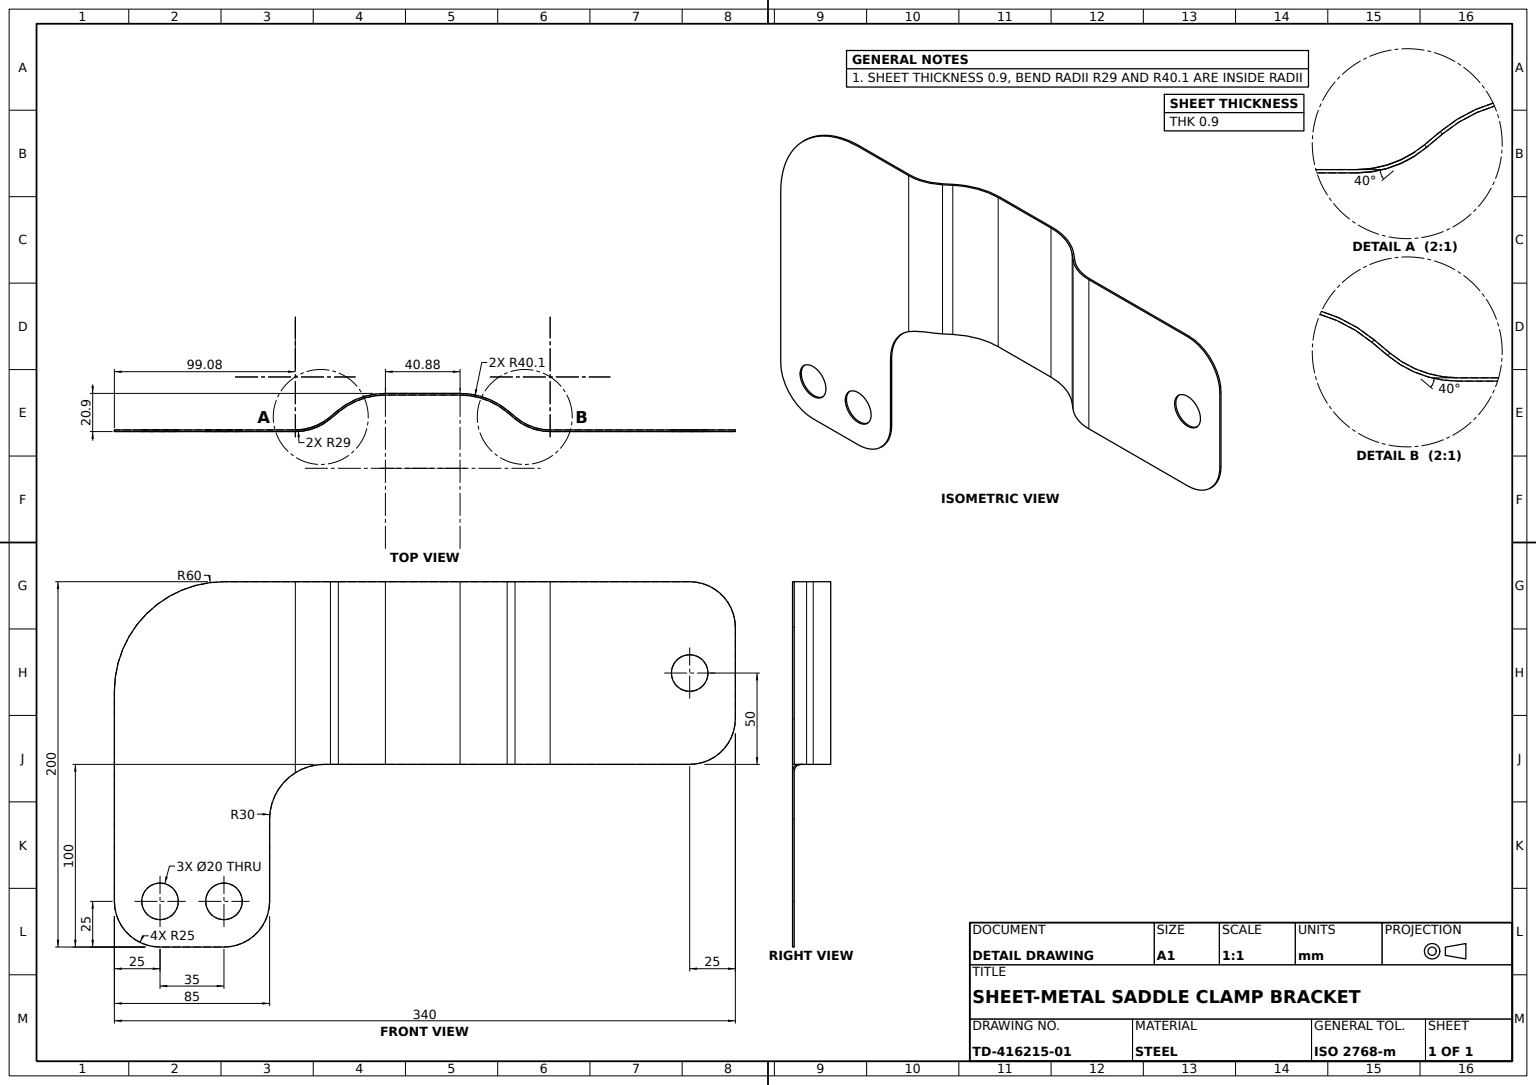
ISO-10303-21;
HEADER;
FILE_DESCRIPTION((''),'2;1');
FILE_NAME('','',(''),(''),'','','');
FILE_SCHEMA(('AUTOMOTIVE_DESIGN'));
ENDSEC;
DATA;
#1=APPLICATION_CONTEXT('');
#2=PRODUCT_CONTEXT('',#1,'mechanical');
#3=PRODUCT('','','',(#2));
#4=PRODUCT_DEFINITION_FORMATION('','',#3);
#5=PRODUCT_DEFINITION_CONTEXT('',#1,'design');
#6=PRODUCT_DEFINITION('','',#4,#5);
#7=PRODUCT_DEFINITION_SHAPE('','',#6);
#8=(LENGTH_UNIT()NAMED_UNIT(*)SI_UNIT(.MILLI.,.METRE.));
#9=(NAMED_UNIT(*)PLANE_ANGLE_UNIT()SI_UNIT($,.RADIAN.));
#10=(NAMED_UNIT(*)SI_UNIT($,.STERADIAN.)SOLID_ANGLE_UNIT());
#11=UNCERTAINTY_MEASURE_WITH_UNIT(LENGTH_MEASURE(1.E-05),#8,'distance_accuracy_value','');
#12=(GEOMETRIC_REPRESENTATION_CONTEXT(3)GLOBAL_UNCERTAINTY_ASSIGNED_CONTEXT((#11))GLOBAL_UNIT_ASSIGNED_CONTEXT((#8,#9,#10))REPRESENTATION_CONTEXT('',''));
#13=CARTESIAN_POINT('',(148.393881,0.,-221.));
#14=VERTEX_POINT('',#13);
#15=CARTESIAN_POINT('',(189.276262,0.,-221.));
#16=VERTEX_POINT('',#15);
#17=DIRECTION('',(1.,0.,0.));
#18=VECTOR('',#17,1000.);
#19=LINE('',#13,#18);
#20=EDGE_CURVE('',#14,#16,#19,.T.);
#21=ORIENTED_EDGE('',*,*,#20,.T.);
#22=CARTESIAN_POINT('',(189.276262,0.,-220.1));
#23=VERTEX_POINT('',#22);
#24=DIRECTION('',(0.,0.,-1.));
#25=VECTOR('',#24,1000.);
#26=LINE('',#15,#25);
#27=EDGE_CURVE('',#23,#16,#26,.T.);
#28=ORIENTED_EDGE('',*,*,#27,.F.);
#29=CARTESIAN_POINT('',(148.393881,0.,-220.1));
#30=VERTEX_POINT('',#29);
#31=LINE('',#29,#18);
#32=EDGE_CURVE('',#30,#23,#31,.T.);
#33=ORIENTED_EDGE('',*,*,#32,.F.);
#34=LINE('',#13,#25);
#35=EDGE_CURVE('',#30,#14,#34,.T.);
#36=ORIENTED_EDGE('',*,*,#35,.T.);
#37=EDGE_LOOP('',(#21,#28,#33,#36));
#38=FACE_OUTER_BOUND('',#37,.T.);
#39=DIRECTION('',(0.,-1.,0.));
#40=AXIS2_PLACEMENT_3D('',#13,#39,#17);
#41=PLANE('',#40);
#42=ADVANCED_FACE('',(#38),#41,.T.);
#43=CARTESIAN_POINT('',(60.,-100.,-201.));
#44=VERTEX_POINT('',#43);
#45=CARTESIAN_POINT('',(60.,-100.,-200.1));
#46=VERTEX_POINT('',#45);
#47=DIRECTION('',(0.,0.,1.));
#48=VECTOR('',#47,1000.);
#49=LINE('',#43,#48);
#50=EDGE_CURVE('',#44,#46,#49,.T.);
#51=ORIENTED_EDGE('',*,*,#50,.F.);
#52=CARTESIAN_POINT('',(85.,-75.,-201.));
#53=VERTEX_POINT('',#52);
#54=CARTESIAN_POINT('',(60.,-75.,-201.));
#55=AXIS2_PLACEMENT_3D('',#54,#24,#17);
#56=CIRCLE('',#55,25.);
#57=EDGE_CURVE('',#53,#44,#56,.T.);
#58=ORIENTED_EDGE('',*,*,#57,.F.);
#59=CARTESIAN_POINT('',(85.,-75.,-200.1));
#60=VERTEX_POINT('',#59);
#61=LINE('',#52,#25);
#62=EDGE_CURVE('',#60,#53,#61,.T.);
#63=ORIENTED_EDGE('',*,*,#62,.F.);
#64=CARTESIAN_POINT('',(60.,-75.,-200.1));
#65=AXIS2_PLACEMENT_3D('',#64,#47,#17);
#66=CIRCLE('',#65,25.);
#67=EDGE_CURVE('',#46,#60,#66,.T.);
#68=ORIENTED_EDGE('',*,*,#67,.F.);
#69=EDGE_LOOP('',(#51,#58,#63,#68));
#70=FACE_OUTER_BOUND('',#69,.T.);
#71=AXIS2_PLACEMENT_3D('',#54,#47,#17);
#72=CYLINDRICAL_SURFACE('',#71,25.);
#73=ADVANCED_FACE('',(#70),#72,.T.);
#74=CARTESIAN_POINT('',(215.052046,100.,-210.718382));
#75=VERTEX_POINT('',#74);
#76=CARTESIAN_POINT('',(215.630554,100.,-211.407822));
#77=VERTEX_POINT('',#76);
#78=DIRECTION('',(0.64278761,0.,-0.766044443));
#79=VECTOR('',#78,1000.);
#80=LINE('',#76,#79);
#81=EDGE_CURVE('',#75,#77,#80,.T.);
#82=ORIENTED_EDGE('',*,*,#81,.T.);
#83=CARTESIAN_POINT('',(189.276262,100.,-221.));
#84=VERTEX_POINT('',#83);
#85=CARTESIAN_POINT('',(189.276262,100.,-180.));
#86=DIRECTION('',(0.,1.,0.));
#87=AXIS2_PLACEMENT_3D('',#85,#86,#24);
#88=CIRCLE('',#87,41.);
#89=EDGE_CURVE('',#77,#84,#88,.T.);
#90=ORIENTED_EDGE('',*,*,#89,.T.);
#91=CARTESIAN_POINT('',(189.276262,100.,-220.1));
#92=VERTEX_POINT('',#91);
#93=LINE('',#83,#25);
#94=EDGE_CURVE('',#92,#84,#93,.T.);
#95=ORIENTED_EDGE('',*,*,#94,.F.);
#96=CIRCLE('',#87,40.1);
#97=EDGE_CURVE('',#75,#92,#96,.T.);
#98=ORIENTED_EDGE('',*,*,#97,.F.);
#99=EDGE_LOOP('',(#82,#90,#95,#98));
#100=FACE_OUTER_BOUND('',#99,.T.);
#101=AXIS2_PLACEMENT_3D('',#85,#86,#47);
#102=PLANE('',#101);
#103=ADVANCED_FACE('',(#100),#102,.T.);
#104=CARTESIAN_POINT('',(25.,-100.,-201.));
#105=VERTEX_POINT('',#104);
#106=CARTESIAN_POINT('',(99.080893,-100.,-201.));
#107=DIRECTION('',(-1.,0.,0.));
#108=VECTOR('',#107,1000.);
#109=LINE('',#106,#108);
#110=EDGE_CURVE('',#44,#105,#109,.T.);
#111=ORIENTED_EDGE('',*,*,#110,.F.);
#112=ORIENTED_EDGE('',*,*,#50,.T.);
#113=CARTESIAN_POINT('',(25.,-100.,-200.1));
#114=VERTEX_POINT('',#113);
#115=CARTESIAN_POINT('',(0.,-100.,-200.1));
#116=LINE('',#115,#108);
#117=EDGE_CURVE('',#46,#114,#116,.T.);
#118=ORIENTED_EDGE('',*,*,#117,.T.);
#119=LINE('',#104,#25);
#120=EDGE_CURVE('',#114,#105,#119,.T.);
#121=ORIENTED_EDGE('',*,*,#120,.T.);
#122=EDGE_LOOP('',(#111,#112,#118,#121));
#123=FACE_OUTER_BOUND('',#122,.T.);
#124=AXIS2_PLACEMENT_3D('',#106,#86,#107);
#125=PLANE('',#124);
#126=ADVANCED_FACE('',(#123),#125,.F.);
#127=CARTESIAN_POINT('',(315.,100.,-200.1));
#128=VERTEX_POINT('',#127);
#129=CARTESIAN_POINT('',(238.589251,100.,-200.1));
#130=VERTEX_POINT('',#129);
#131=LINE('',#129,#108);
#132=EDGE_CURVE('',#128,#130,#131,.T.);
#133=ORIENTED_EDGE('',*,*,#132,.T.);
#134=CARTESIAN_POINT('',(238.589251,0.,-200.1));
#135=VERTEX_POINT('',#134);
#136=VECTOR('',#39,1000.);
#137=LINE('',#129,#136);
#138=EDGE_CURVE('',#130,#135,#137,.T.);
#139=ORIENTED_EDGE('',*,*,#138,.T.);
#140=CARTESIAN_POINT('',(315.,0.,-200.1));
#141=VERTEX_POINT('',#140);
#142=LINE('',#134,#18);
#143=EDGE_CURVE('',#135,#141,#142,.T.);
#144=ORIENTED_EDGE('',*,*,#143,.T.);
#145=CARTESIAN_POINT('',(340.,25.,-200.1));
#146=VERTEX_POINT('',#145);
#147=CARTESIAN_POINT('',(315.,25.,-200.1));
#148=AXIS2_PLACEMENT_3D('',#147,#47,#17);
#149=CIRCLE('',#148,25.);
#150=EDGE_CURVE('',#141,#146,#149,.T.);
#151=ORIENTED_EDGE('',*,*,#150,.T.);
#152=CARTESIAN_POINT('',(340.,75.,-200.1));
#153=VERTEX_POINT('',#152);
#154=CARTESIAN_POINT('',(340.,100.,-200.1));
#155=LINE('',#154,#136);
#156=EDGE_CURVE('',#153,#146,#155,.T.);
#157=ORIENTED_EDGE('',*,*,#156,.F.);
#158=CARTESIAN_POINT('',(315.,75.,-200.1));
#159=AXIS2_PLACEMENT_3D('',#158,#47,#17);
#160=CIRCLE('',#159,25.);
#161=EDGE_CURVE('',#153,#128,#160,.T.);
#162=ORIENTED_EDGE('',*,*,#161,.T.);
#163=EDGE_LOOP('',(#133,#139,#144,#151,#157,#162));
#164=FACE_OUTER_BOUND('',#163,.T.);
#165=CARTESIAN_POINT('',(325.,50.,-200.1));
#166=VERTEX_POINT('',#165);
#167=CARTESIAN_POINT('',(305.,50.,-200.1));
#168=VERTEX_POINT('',#167);
#169=CARTESIAN_POINT('',(315.,50.,-200.1));
#170=AXIS2_PLACEMENT_3D('',#169,#47,#17);
#171=CIRCLE('',#170,10.);
#172=EDGE_CURVE('',#166,#168,#171,.T.);
#173=ORIENTED_EDGE('',*,*,#172,.F.);
#174=EDGE_CURVE('',#168,#166,#171,.T.);
#175=ORIENTED_EDGE('',*,*,#174,.F.);
#176=EDGE_LOOP('',(#173,#175));
#177=FACE_BOUND('',#176,.T.);
#178=AXIS2_PLACEMENT_3D('',#129,#47,#17);
#179=PLANE('',#178);
#180=ADVANCED_FACE('',(#164,#177),#179,.T.);
#181=CARTESIAN_POINT('',(305.,50.,-201.));
#182=VERTEX_POINT('',#181);
#183=CARTESIAN_POINT('',(305.,50.,44.));
#184=LINE('',#183,#25);
#185=EDGE_CURVE('',#168,#182,#184,.T.);
#186=ORIENTED_EDGE('',*,*,#185,.F.);
#187=ORIENTED_EDGE('',*,*,#174,.T.);
#188=CARTESIAN_POINT('',(325.,50.,-201.));
#189=VERTEX_POINT('',#188);
#190=CARTESIAN_POINT('',(325.,50.,44.));
#191=LINE('',#190,#25);
#192=EDGE_CURVE('',#166,#189,#191,.T.);
#193=ORIENTED_EDGE('',*,*,#192,.T.);
#194=CARTESIAN_POINT('',(315.,50.,-201.));
#195=AXIS2_PLACEMENT_3D('',#194,#24,#107);
#196=CIRCLE('',#195,10.);
#197=EDGE_CURVE('',#189,#182,#196,.T.);
#198=ORIENTED_EDGE('',*,*,#197,.T.);
#199=EDGE_LOOP('',(#186,#187,#193,#198));
#200=FACE_OUTER_BOUND('',#199,.T.);
#201=CARTESIAN_POINT('',(315.,50.,44.));
#202=AXIS2_PLACEMENT_3D('',#201,#24,#107);
#203=CYLINDRICAL_SURFACE('',#202,10.);
#204=ADVANCED_FACE('',(#200),#203,.F.);
#205=CARTESIAN_POINT('',(219.369901,0.,-207.095271));
#206=VERTEX_POINT('',#205);
#207=CARTESIAN_POINT('',(219.94841,0.,-207.784711));
#208=VERTEX_POINT('',#207);
#209=LINE('',#207,#79);
#210=EDGE_CURVE('',#206,#208,#209,.T.);
#211=ORIENTED_EDGE('',*,*,#210,.F.);
#212=CARTESIAN_POINT('',(215.052046,0.,-210.718382));
#213=VERTEX_POINT('',#212);
#214=DIRECTION('',(0.766044443,0.,0.64278761));
#215=VECTOR('',#214,1000.);
#216=LINE('',#212,#215);
#217=EDGE_CURVE('',#213,#206,#216,.T.);
#218=ORIENTED_EDGE('',*,*,#217,.F.);
#219=CARTESIAN_POINT('',(215.630554,0.,-211.407822));
#220=VERTEX_POINT('',#219);
#221=LINE('',#219,#79);
#222=EDGE_CURVE('',#213,#220,#221,.T.);
#223=ORIENTED_EDGE('',*,*,#222,.T.);
#224=LINE('',#219,#215);
#225=EDGE_CURVE('',#220,#208,#224,.T.);
#226=ORIENTED_EDGE('',*,*,#225,.T.);
#227=EDGE_LOOP('',(#211,#218,#223,#226));
#228=FACE_OUTER_BOUND('',#227,.T.);
#229=AXIS2_PLACEMENT_3D('',#219,#39,#214);
#230=PLANE('',#229);
#231=ADVANCED_FACE('',(#228),#230,.T.);
#232=CARTESIAN_POINT('',(0.,40.,-200.1));
#233=VERTEX_POINT('',#232);
#234=CARTESIAN_POINT('',(0.,40.,-201.));
#235=VERTEX_POINT('',#234);
#236=LINE('',#234,#25);
#237=EDGE_CURVE('',#233,#235,#236,.T.);
#238=ORIENTED_EDGE('',*,*,#237,.F.);
#239=CARTESIAN_POINT('',(60.,100.,-200.1));
#240=VERTEX_POINT('',#239);
#241=CARTESIAN_POINT('',(60.,40.,-200.1));
#242=AXIS2_PLACEMENT_3D('',#241,#47,#17);
#243=CIRCLE('',#242,60.);
#244=EDGE_CURVE('',#240,#233,#243,.T.);
#245=ORIENTED_EDGE('',*,*,#244,.F.);
#246=CARTESIAN_POINT('',(60.,100.,-201.));
#247=VERTEX_POINT('',#246);
#248=LINE('',#246,#48);
#249=EDGE_CURVE('',#247,#240,#248,.T.);
#250=ORIENTED_EDGE('',*,*,#249,.F.);
#251=CARTESIAN_POINT('',(60.,40.,-201.));
#252=AXIS2_PLACEMENT_3D('',#251,#24,#17);
#253=CIRCLE('',#252,60.);
#254=EDGE_CURVE('',#235,#247,#253,.T.);
#255=ORIENTED_EDGE('',*,*,#254,.F.);
#256=EDGE_LOOP('',(#238,#245,#250,#255));
#257=FACE_OUTER_BOUND('',#256,.T.);
#258=AXIS2_PLACEMENT_3D('',#251,#24,#107);
#259=CYLINDRICAL_SURFACE('',#258,60.);
#260=ADVANCED_FACE('',(#257),#259,.T.);
#261=CARTESIAN_POINT('',(118.300243,100.,-207.095271));
#262=VERTEX_POINT('',#261);
#263=CARTESIAN_POINT('',(118.300243,0.,-207.095271));
#264=VERTEX_POINT('',#263);
#265=LINE('',#261,#136);
#266=EDGE_CURVE('',#262,#264,#265,.T.);
#267=ORIENTED_EDGE('',*,*,#266,.T.);
#268=CARTESIAN_POINT('',(122.618098,0.,-210.718382));
#269=VERTEX_POINT('',#268);
#270=DIRECTION('',(0.766044443,0.,-0.64278761));
#271=VECTOR('',#270,1000.);
#272=LINE('',#263,#271);
#273=EDGE_CURVE('',#264,#269,#272,.T.);
#274=ORIENTED_EDGE('',*,*,#273,.T.);
#275=CARTESIAN_POINT('',(122.618098,100.,-210.718382));
#276=VERTEX_POINT('',#275);
#277=LINE('',#275,#136);
#278=EDGE_CURVE('',#276,#269,#277,.T.);
#279=ORIENTED_EDGE('',*,*,#278,.F.);
#280=DIRECTION('',(-0.766044443,0.,0.64278761));
#281=VECTOR('',#280,1000.);
#282=LINE('',#261,#281);
#283=EDGE_CURVE('',#276,#262,#282,.T.);
#284=ORIENTED_EDGE('',*,*,#283,.T.);
#285=EDGE_LOOP('',(#267,#274,#279,#284));
#286=FACE_OUTER_BOUND('',#285,.T.);
#287=DIRECTION('',(0.64278761,0.,0.766044443));
#288=AXIS2_PLACEMENT_3D('',#261,#287,#270);
#289=PLANE('',#288);
#290=ADVANCED_FACE('',(#286),#289,.T.);
#291=ORIENTED_EDGE('',*,*,#225,.F.);
#292=LINE('',#76,#136);
#293=EDGE_CURVE('',#77,#220,#292,.T.);
#294=ORIENTED_EDGE('',*,*,#293,.F.);
#295=CARTESIAN_POINT('',(219.94841,100.,-207.784711));
#296=VERTEX_POINT('',#295);
#297=CARTESIAN_POINT('',(138.081545,100.,-276.479167));
#298=DIRECTION('',(-0.766044443,0.,-0.64278761));
#299=VECTOR('',#298,1000.);
#300=LINE('',#297,#299);
#301=EDGE_CURVE('',#296,#77,#300,.T.);
#302=ORIENTED_EDGE('',*,*,#301,.F.);
#303=LINE('',#295,#136);
#304=EDGE_CURVE('',#296,#208,#303,.T.);
#305=ORIENTED_EDGE('',*,*,#304,.T.);
#306=EDGE_LOOP('',(#291,#294,#302,#305));
#307=FACE_OUTER_BOUND('',#306,.T.);
#308=DIRECTION('',(-0.64278761,0.,0.766044443));
#309=AXIS2_PLACEMENT_3D('',#76,#308,#214);
#310=PLANE('',#309);
#311=ADVANCED_FACE('',(#307),#310,.F.);
#312=CARTESIAN_POINT('',(315.,100.,-201.));
#313=VERTEX_POINT('',#312);
#314=LINE('',#312,#25);
#315=EDGE_CURVE('',#128,#313,#314,.T.);
#316=ORIENTED_EDGE('',*,*,#315,.F.);
#317=ORIENTED_EDGE('',*,*,#161,.F.);
#318=CARTESIAN_POINT('',(340.,75.,-201.));
#319=VERTEX_POINT('',#318);
#320=LINE('',#318,#48);
#321=EDGE_CURVE('',#319,#153,#320,.T.);
#322=ORIENTED_EDGE('',*,*,#321,.F.);
#323=CARTESIAN_POINT('',(315.,75.,-201.));
#324=AXIS2_PLACEMENT_3D('',#323,#24,#17);
#325=CIRCLE('',#324,25.);
#326=EDGE_CURVE('',#313,#319,#325,.T.);
#327=ORIENTED_EDGE('',*,*,#326,.F.);
#328=EDGE_LOOP('',(#316,#317,#322,#327));
#329=FACE_OUTER_BOUND('',#328,.T.);
#330=AXIS2_PLACEMENT_3D('',#323,#47,#17);
#331=CYLINDRICAL_SURFACE('',#330,25.);
#332=ADVANCED_FACE('',(#329),#331,.T.);
#333=CARTESIAN_POINT('',(238.589251,0.,-230.));
#334=AXIS2_PLACEMENT_3D('',#333,#86,#24);
#335=CIRCLE('',#334,29.9);
#336=EDGE_CURVE('',#206,#135,#335,.T.);
#337=ORIENTED_EDGE('',*,*,#336,.F.);
#338=ORIENTED_EDGE('',*,*,#210,.T.);
#339=CARTESIAN_POINT('',(238.589251,0.,-201.));
#340=VERTEX_POINT('',#339);
#341=AXIS2_PLACEMENT_3D('',#333,#86,#17);
#342=CIRCLE('',#341,29.);
#343=EDGE_CURVE('',#208,#340,#342,.T.);
#344=ORIENTED_EDGE('',*,*,#343,.T.);
#345=LINE('',#339,#25);
#346=EDGE_CURVE('',#135,#340,#345,.T.);
#347=ORIENTED_EDGE('',*,*,#346,.F.);
#348=EDGE_LOOP('',(#337,#338,#344,#347));
#349=FACE_OUTER_BOUND('',#348,.T.);
#350=AXIS2_PLACEMENT_3D('',#333,#86,#107);
#351=PLANE('',#350);
#352=ADVANCED_FACE('',(#349),#351,.F.);
#353=CARTESIAN_POINT('',(340.,25.,-201.));
#354=VERTEX_POINT('',#353);
#355=CARTESIAN_POINT('',(315.,0.,-201.));
#356=VERTEX_POINT('',#355);
#357=CARTESIAN_POINT('',(315.,25.,-201.));
#358=AXIS2_PLACEMENT_3D('',#357,#24,#17);
#359=CIRCLE('',#358,25.);
#360=EDGE_CURVE('',#354,#356,#359,.T.);
#361=ORIENTED_EDGE('',*,*,#360,.F.);
#362=LINE('',#353,#25);
#363=EDGE_CURVE('',#146,#354,#362,.T.);
#364=ORIENTED_EDGE('',*,*,#363,.F.);
#365=ORIENTED_EDGE('',*,*,#150,.F.);
#366=LINE('',#355,#48);
#367=EDGE_CURVE('',#356,#141,#366,.T.);
#368=ORIENTED_EDGE('',*,*,#367,.F.);
#369=EDGE_LOOP('',(#361,#364,#365,#368));
#370=FACE_OUTER_BOUND('',#369,.T.);
#371=AXIS2_PLACEMENT_3D('',#357,#47,#17);
#372=CYLINDRICAL_SURFACE('',#371,25.);
#373=ADVANCED_FACE('',(#370),#372,.T.);
#374=CARTESIAN_POINT('',(148.393881,100.,-221.));
#375=VERTEX_POINT('',#374);
#376=LINE('',#374,#136);
#377=EDGE_CURVE('',#375,#14,#376,.T.);
#378=ORIENTED_EDGE('',*,*,#377,.F.);
#379=CARTESIAN_POINT('',(99.080893,100.,-221.));
#380=LINE('',#379,#108);
#381=EDGE_CURVE('',#84,#375,#380,.T.);
#382=ORIENTED_EDGE('',*,*,#381,.F.);
#383=LINE('',#83,#136);
#384=EDGE_CURVE('',#84,#16,#383,.T.);
#385=ORIENTED_EDGE('',*,*,#384,.T.);
#386=ORIENTED_EDGE('',*,*,#20,.F.);
#387=EDGE_LOOP('',(#378,#382,#385,#386));
#388=FACE_OUTER_BOUND('',#387,.T.);
#389=AXIS2_PLACEMENT_3D('',#374,#47,#17);
#390=PLANE('',#389);
#391=ADVANCED_FACE('',(#388),#390,.F.);
#392=CARTESIAN_POINT('',(219.369901,100.,-207.095271));
#393=VERTEX_POINT('',#392);
#394=LINE('',#295,#79);
#395=EDGE_CURVE('',#393,#296,#394,.T.);
#396=ORIENTED_EDGE('',*,*,#395,.T.);
#397=ORIENTED_EDGE('',*,*,#301,.T.);
#398=ORIENTED_EDGE('',*,*,#81,.F.);
#399=LINE('',#74,#299);
#400=EDGE_CURVE('',#393,#75,#399,.T.);
#401=ORIENTED_EDGE('',*,*,#400,.F.);
#402=EDGE_LOOP('',(#396,#397,#398,#401));
#403=FACE_OUTER_BOUND('',#402,.T.);
#404=AXIS2_PLACEMENT_3D('',#297,#86,#298);
#405=PLANE('',#404);
#406=ADVANCED_FACE('',(#403),#405,.T.);
#407=CARTESIAN_POINT('',(0.,-75.,-201.));
#408=VERTEX_POINT('',#407);
#409=CARTESIAN_POINT('',(25.,-75.,-201.));
#410=AXIS2_PLACEMENT_3D('',#409,#24,#17);
#411=CIRCLE('',#410,25.);
#412=EDGE_CURVE('',#105,#408,#411,.T.);
#413=ORIENTED_EDGE('',*,*,#412,.T.);
#414=CARTESIAN_POINT('',(0.,100.,-201.));
#415=LINE('',#414,#136);
#416=EDGE_CURVE('',#235,#408,#415,.T.);
#417=ORIENTED_EDGE('',*,*,#416,.F.);
#418=ORIENTED_EDGE('',*,*,#254,.T.);
#419=CARTESIAN_POINT('',(99.080893,100.,-201.));
#420=VERTEX_POINT('',#419);
#421=LINE('',#419,#108);
#422=EDGE_CURVE('',#420,#247,#421,.T.);
#423=ORIENTED_EDGE('',*,*,#422,.F.);
#424=CARTESIAN_POINT('',(99.080893,-4.572023,-201.));
#425=VERTEX_POINT('',#424);
#426=LINE('',#419,#136);
#427=EDGE_CURVE('',#420,#425,#426,.T.);
#428=ORIENTED_EDGE('',*,*,#427,.T.);
#429=CARTESIAN_POINT('',(85.,-30.,-201.));
#430=VERTEX_POINT('',#429);
#431=CARTESIAN_POINT('',(115.,-30.,-201.));
#432=AXIS2_PLACEMENT_3D('',#431,#47,#17);
#433=CIRCLE('',#432,30.);
#434=EDGE_CURVE('',#425,#430,#433,.T.);
#435=ORIENTED_EDGE('',*,*,#434,.T.);
#436=CARTESIAN_POINT('',(85.,100.,-201.));
#437=VECTOR('',#86,1000.);
#438=LINE('',#436,#437);
#439=EDGE_CURVE('',#53,#430,#438,.T.);
#440=ORIENTED_EDGE('',*,*,#439,.F.);
#441=ORIENTED_EDGE('',*,*,#57,.T.);
#442=ORIENTED_EDGE('',*,*,#110,.T.);
#443=EDGE_LOOP('',(#413,#417,#418,#423,#428,#435,#440,#441,#442));
#444=FACE_OUTER_BOUND('',#443,.T.);
#445=CARTESIAN_POINT('',(35.,-75.,-201.));
#446=VERTEX_POINT('',#445);
#447=CARTESIAN_POINT('',(15.,-75.,-201.));
#448=VERTEX_POINT('',#447);
#449=AXIS2_PLACEMENT_3D('',#409,#24,#107);
#450=CIRCLE('',#449,10.);
#451=EDGE_CURVE('',#446,#448,#450,.T.);
#452=ORIENTED_EDGE('',*,*,#451,.F.);
#453=EDGE_CURVE('',#448,#446,#450,.T.);
#454=ORIENTED_EDGE('',*,*,#453,.F.);
#455=EDGE_LOOP('',(#452,#454));
#456=FACE_BOUND('',#455,.T.);
#457=CARTESIAN_POINT('',(50.,-75.,-201.));
#458=VERTEX_POINT('',#457);
#459=CARTESIAN_POINT('',(70.,-75.,-201.));
#460=VERTEX_POINT('',#459);
#461=AXIS2_PLACEMENT_3D('',#54,#24,#107);
#462=CIRCLE('',#461,10.);
#463=EDGE_CURVE('',#458,#460,#462,.T.);
#464=ORIENTED_EDGE('',*,*,#463,.F.);
#465=EDGE_CURVE('',#460,#458,#462,.T.);
#466=ORIENTED_EDGE('',*,*,#465,.F.);
#467=EDGE_LOOP('',(#464,#466));
#468=FACE_BOUND('',#467,.T.);
#469=AXIS2_PLACEMENT_3D('',#414,#47,#17);
#470=PLANE('',#469);
#471=ADVANCED_FACE('',(#444,#456,#468),#470,.F.);
#472=ORIENTED_EDGE('',*,*,#384,.F.);
#473=ORIENTED_EDGE('',*,*,#89,.F.);
#474=ORIENTED_EDGE('',*,*,#293,.T.);
#475=CARTESIAN_POINT('',(189.276262,0.,-180.));
#476=AXIS2_PLACEMENT_3D('',#475,#39,#17);
#477=CIRCLE('',#476,41.);
#478=EDGE_CURVE('',#16,#220,#477,.T.);
#479=ORIENTED_EDGE('',*,*,#478,.F.);
#480=EDGE_LOOP('',(#472,#473,#474,#479));
#481=FACE_OUTER_BOUND('',#480,.T.);
#482=AXIS2_PLACEMENT_3D('',#85,#39,#24);
#483=CYLINDRICAL_SURFACE('',#482,41.);
#484=ADVANCED_FACE('',(#481),#483,.T.);
#485=ORIENTED_EDGE('',*,*,#27,.T.);
#486=ORIENTED_EDGE('',*,*,#478,.T.);
#487=ORIENTED_EDGE('',*,*,#222,.F.);
#488=AXIS2_PLACEMENT_3D('',#475,#39,#24);
#489=CIRCLE('',#488,40.1);
#490=EDGE_CURVE('',#23,#213,#489,.T.);
#491=ORIENTED_EDGE('',*,*,#490,.F.);
#492=EDGE_LOOP('',(#485,#486,#487,#491));
#493=FACE_OUTER_BOUND('',#492,.T.);
#494=AXIS2_PLACEMENT_3D('',#475,#86,#107);
#495=PLANE('',#494);
#496=ADVANCED_FACE('',(#493),#495,.F.);
#497=EDGE_CURVE('',#182,#189,#196,.T.);
#498=ORIENTED_EDGE('',*,*,#497,.F.);
#499=ORIENTED_EDGE('',*,*,#197,.F.);
#500=EDGE_LOOP('',(#498,#499));
#501=FACE_BOUND('',#500,.T.);
#502=ORIENTED_EDGE('',*,*,#360,.T.);
#503=LINE('',#339,#18);
#504=EDGE_CURVE('',#340,#356,#503,.T.);
#505=ORIENTED_EDGE('',*,*,#504,.F.);
#506=CARTESIAN_POINT('',(238.589251,100.,-201.));
#507=VERTEX_POINT('',#506);
#508=LINE('',#506,#136);
#509=EDGE_CURVE('',#507,#340,#508,.T.);
#510=ORIENTED_EDGE('',*,*,#509,.F.);
#511=EDGE_CURVE('',#313,#507,#421,.T.);
#512=ORIENTED_EDGE('',*,*,#511,.F.);
#513=ORIENTED_EDGE('',*,*,#326,.T.);
#514=CARTESIAN_POINT('',(340.,100.,-201.));
#515=LINE('',#514,#136);
#516=EDGE_CURVE('',#319,#354,#515,.T.);
#517=ORIENTED_EDGE('',*,*,#516,.T.);
#518=EDGE_LOOP('',(#502,#505,#510,#512,#513,#517));
#519=FACE_OUTER_BOUND('',#518,.T.);
#520=AXIS2_PLACEMENT_3D('',#506,#47,#17);
#521=PLANE('',#520);
#522=ADVANCED_FACE('',(#501,#519),#521,.F.);
#523=CARTESIAN_POINT('',(99.080893,100.,-200.1));
#524=VERTEX_POINT('',#523);
#525=LINE('',#419,#25);
#526=EDGE_CURVE('',#524,#420,#525,.T.);
#527=ORIENTED_EDGE('',*,*,#526,.F.);
#528=CARTESIAN_POINT('',(99.080893,100.,-230.));
#529=AXIS2_PLACEMENT_3D('',#528,#39,#24);
#530=CIRCLE('',#529,29.9);
#531=EDGE_CURVE('',#262,#524,#530,.T.);
#532=ORIENTED_EDGE('',*,*,#531,.F.);
#533=CARTESIAN_POINT('',(117.721734,100.,-207.784711));
#534=VERTEX_POINT('',#533);
#535=DIRECTION('',(-0.64278761,0.,-0.766044443));
#536=VECTOR('',#535,1000.);
#537=LINE('',#533,#536);
#538=EDGE_CURVE('',#262,#534,#537,.T.);
#539=ORIENTED_EDGE('',*,*,#538,.T.);
#540=CIRCLE('',#529,29.);
#541=EDGE_CURVE('',#534,#420,#540,.T.);
#542=ORIENTED_EDGE('',*,*,#541,.T.);
#543=EDGE_LOOP('',(#527,#532,#539,#542));
#544=FACE_OUTER_BOUND('',#543,.T.);
#545=AXIS2_PLACEMENT_3D('',#528,#86,#47);
#546=PLANE('',#545);
#547=ADVANCED_FACE('',(#544),#546,.T.);
#548=ORIENTED_EDGE('',*,*,#363,.T.);
#549=ORIENTED_EDGE('',*,*,#516,.F.);
#550=ORIENTED_EDGE('',*,*,#321,.T.);
#551=ORIENTED_EDGE('',*,*,#156,.T.);
#552=EDGE_LOOP('',(#548,#549,#550,#551));
#553=FACE_OUTER_BOUND('',#552,.T.);
#554=AXIS2_PLACEMENT_3D('',#514,#107,#39);
#555=PLANE('',#554);
#556=ADVANCED_FACE('',(#553),#555,.F.);
#557=ORIENTED_EDGE('',*,*,#138,.F.);
#558=CARTESIAN_POINT('',(238.589251,100.,-230.));
#559=AXIS2_PLACEMENT_3D('',#558,#39,#24);
#560=CIRCLE('',#559,29.9);
#561=EDGE_CURVE('',#130,#393,#560,.T.);
#562=ORIENTED_EDGE('',*,*,#561,.T.);
#563=LINE('',#392,#136);
#564=EDGE_CURVE('',#393,#206,#563,.T.);
#565=ORIENTED_EDGE('',*,*,#564,.T.);
#566=ORIENTED_EDGE('',*,*,#336,.T.);
#567=EDGE_LOOP('',(#557,#562,#565,#566));
#568=FACE_OUTER_BOUND('',#567,.T.);
#569=CYLINDRICAL_SURFACE('',#559,29.9);
#570=ADVANCED_FACE('',(#568),#569,.T.);
#571=CARTESIAN_POINT('',(122.039589,100.,-211.407822));
#572=VERTEX_POINT('',#571);
#573=LINE('',#533,#281);
#574=EDGE_CURVE('',#572,#534,#573,.T.);
#575=ORIENTED_EDGE('',*,*,#574,.T.);
#576=ORIENTED_EDGE('',*,*,#538,.F.);
#577=ORIENTED_EDGE('',*,*,#283,.F.);
#578=LINE('',#571,#536);
#579=EDGE_CURVE('',#276,#572,#578,.T.);
#580=ORIENTED_EDGE('',*,*,#579,.T.);
#581=EDGE_LOOP('',(#575,#576,#577,#580));
#582=FACE_OUTER_BOUND('',#581,.T.);
#583=AXIS2_PLACEMENT_3D('',#533,#86,#280);
#584=PLANE('',#583);
#585=ADVANCED_FACE('',(#582),#584,.T.);
#586=ORIENTED_EDGE('',*,*,#511,.T.);
#587=LINE('',#506,#25);
#588=EDGE_CURVE('',#130,#507,#587,.T.);
#589=ORIENTED_EDGE('',*,*,#588,.F.);
#590=ORIENTED_EDGE('',*,*,#132,.F.);
#591=ORIENTED_EDGE('',*,*,#315,.T.);
#592=EDGE_LOOP('',(#586,#589,#590,#591));
#593=FACE_OUTER_BOUND('',#592,.T.);
#594=AXIS2_PLACEMENT_3D('',#419,#86,#107);
#595=PLANE('',#594);
#596=ADVANCED_FACE('',(#593),#595,.T.);
#597=CARTESIAN_POINT('',(122.039589,0.,-211.407822));
#598=VERTEX_POINT('',#597);
#599=LINE('',#597,#536);
#600=EDGE_CURVE('',#269,#598,#599,.T.);
#601=ORIENTED_EDGE('',*,*,#600,.F.);
#602=ORIENTED_EDGE('',*,*,#273,.F.);
#603=CARTESIAN_POINT('',(117.721734,0.,-207.784711));
#604=VERTEX_POINT('',#603);
#605=LINE('',#603,#536);
#606=EDGE_CURVE('',#264,#604,#605,.T.);
#607=ORIENTED_EDGE('',*,*,#606,.T.);
#608=LINE('',#603,#271);
#609=EDGE_CURVE('',#604,#598,#608,.T.);
#610=ORIENTED_EDGE('',*,*,#609,.T.);
#611=EDGE_LOOP('',(#601,#602,#607,#610));
#612=FACE_OUTER_BOUND('',#611,.T.);
#613=AXIS2_PLACEMENT_3D('',#603,#39,#270);
#614=PLANE('',#613);
#615=ADVANCED_FACE('',(#612),#614,.T.);
#616=LINE('',#91,#136);
#617=EDGE_CURVE('',#92,#23,#616,.T.);
#618=ORIENTED_EDGE('',*,*,#617,.T.);
#619=ORIENTED_EDGE('',*,*,#490,.T.);
#620=LINE('',#74,#136);
#621=EDGE_CURVE('',#75,#213,#620,.T.);
#622=ORIENTED_EDGE('',*,*,#621,.F.);
#623=ORIENTED_EDGE('',*,*,#97,.T.);
#624=EDGE_LOOP('',(#618,#619,#622,#623));
#625=FACE_OUTER_BOUND('',#624,.T.);
#626=CYLINDRICAL_SURFACE('',#482,40.1);
#627=ADVANCED_FACE('',(#625),#626,.F.);
#628=CARTESIAN_POINT('',(148.393881,0.,-180.));
#629=AXIS2_PLACEMENT_3D('',#628,#39,#17);
#630=CIRCLE('',#629,41.);
#631=EDGE_CURVE('',#598,#14,#630,.T.);
#632=ORIENTED_EDGE('',*,*,#631,.F.);
#633=LINE('',#571,#136);
#634=EDGE_CURVE('',#572,#598,#633,.T.);
#635=ORIENTED_EDGE('',*,*,#634,.F.);
#636=CARTESIAN_POINT('',(148.393881,100.,-180.));
#637=AXIS2_PLACEMENT_3D('',#636,#86,#24);
#638=CIRCLE('',#637,41.);
#639=EDGE_CURVE('',#375,#572,#638,.T.);
#640=ORIENTED_EDGE('',*,*,#639,.F.);
#641=ORIENTED_EDGE('',*,*,#377,.T.);
#642=EDGE_LOOP('',(#632,#635,#640,#641));
#643=FACE_OUTER_BOUND('',#642,.T.);
#644=AXIS2_PLACEMENT_3D('',#636,#39,#24);
#645=CYLINDRICAL_SURFACE('',#644,41.);
#646=ADVANCED_FACE('',(#643),#645,.T.);
#647=CARTESIAN_POINT('',(35.,-75.,-200.1));
#648=VERTEX_POINT('',#647);
#649=CARTESIAN_POINT('',(35.,-75.,44.));
#650=LINE('',#649,#25);
#651=EDGE_CURVE('',#648,#446,#650,.T.);
#652=ORIENTED_EDGE('',*,*,#651,.T.);
#653=ORIENTED_EDGE('',*,*,#451,.T.);
#654=CARTESIAN_POINT('',(15.,-75.,-200.1));
#655=VERTEX_POINT('',#654);
#656=CARTESIAN_POINT('',(15.,-75.,44.));
#657=LINE('',#656,#25);
#658=EDGE_CURVE('',#655,#448,#657,.T.);
#659=ORIENTED_EDGE('',*,*,#658,.F.);
#660=CARTESIAN_POINT('',(25.,-75.,-200.1));
#661=AXIS2_PLACEMENT_3D('',#660,#47,#17);
#662=CIRCLE('',#661,10.);
#663=EDGE_CURVE('',#655,#648,#662,.T.);
#664=ORIENTED_EDGE('',*,*,#663,.T.);
#665=EDGE_LOOP('',(#652,#653,#659,#664));
#666=FACE_OUTER_BOUND('',#665,.T.);
#667=CARTESIAN_POINT('',(25.,-75.,44.));
#668=AXIS2_PLACEMENT_3D('',#667,#24,#107);
#669=CYLINDRICAL_SURFACE('',#668,10.);
#670=ADVANCED_FACE('',(#666),#669,.F.);
#671=ORIENTED_EDGE('',*,*,#304,.F.);
#672=CIRCLE('',#559,29.);
#673=EDGE_CURVE('',#507,#296,#672,.T.);
#674=ORIENTED_EDGE('',*,*,#673,.F.);
#675=ORIENTED_EDGE('',*,*,#509,.T.);
#676=ORIENTED_EDGE('',*,*,#343,.F.);
#677=EDGE_LOOP('',(#671,#674,#675,#676));
#678=FACE_OUTER_BOUND('',#677,.T.);
#679=CYLINDRICAL_SURFACE('',#559,29.);
#680=ADVANCED_FACE('',(#678),#679,.F.);
#681=EDGE_CURVE('',#648,#655,#662,.T.);
#682=ORIENTED_EDGE('',*,*,#681,.F.);
#683=ORIENTED_EDGE('',*,*,#663,.F.);
#684=EDGE_LOOP('',(#682,#683));
#685=FACE_BOUND('',#684,.T.);
#686=ORIENTED_EDGE('',*,*,#117,.F.);
#687=ORIENTED_EDGE('',*,*,#67,.T.);
#688=CARTESIAN_POINT('',(85.,-30.,-200.1));
#689=VERTEX_POINT('',#688);
#690=CARTESIAN_POINT('',(85.,100.,-200.1));
#691=LINE('',#690,#437);
#692=EDGE_CURVE('',#60,#689,#691,.T.);
#693=ORIENTED_EDGE('',*,*,#692,.T.);
#694=CARTESIAN_POINT('',(99.080893,-4.572023,-200.1));
#695=VERTEX_POINT('',#694);
#696=CARTESIAN_POINT('',(115.,-30.,-200.1));
#697=AXIS2_PLACEMENT_3D('',#696,#24,#17);
#698=CIRCLE('',#697,30.);
#699=EDGE_CURVE('',#689,#695,#698,.T.);
#700=ORIENTED_EDGE('',*,*,#699,.T.);
#701=LINE('',#523,#136);
#702=EDGE_CURVE('',#524,#695,#701,.T.);
#703=ORIENTED_EDGE('',*,*,#702,.F.);
#704=CARTESIAN_POINT('',(0.,100.,-200.1));
#705=LINE('',#704,#108);
#706=EDGE_CURVE('',#524,#240,#705,.T.);
#707=ORIENTED_EDGE('',*,*,#706,.T.);
#708=ORIENTED_EDGE('',*,*,#244,.T.);
#709=CARTESIAN_POINT('',(0.,-75.,-200.1));
#710=VERTEX_POINT('',#709);
#711=LINE('',#704,#136);
#712=EDGE_CURVE('',#233,#710,#711,.T.);
#713=ORIENTED_EDGE('',*,*,#712,.T.);
#714=CIRCLE('',#661,25.);
#715=EDGE_CURVE('',#710,#114,#714,.T.);
#716=ORIENTED_EDGE('',*,*,#715,.T.);
#717=EDGE_LOOP('',(#686,#687,#693,#700,#703,#707,#708,#713,#716));
#718=FACE_OUTER_BOUND('',#717,.T.);
#719=CARTESIAN_POINT('',(50.,-75.,-200.1));
#720=VERTEX_POINT('',#719);
#721=CARTESIAN_POINT('',(70.,-75.,-200.1));
#722=VERTEX_POINT('',#721);
#723=CIRCLE('',#65,10.);
#724=EDGE_CURVE('',#720,#722,#723,.T.);
#725=ORIENTED_EDGE('',*,*,#724,.F.);
#726=EDGE_CURVE('',#722,#720,#723,.T.);
#727=ORIENTED_EDGE('',*,*,#726,.F.);
#728=EDGE_LOOP('',(#725,#727));
#729=FACE_BOUND('',#728,.T.);
#730=AXIS2_PLACEMENT_3D('',#704,#47,#17);
#731=PLANE('',#730);
#732=ADVANCED_FACE('',(#685,#718,#729),#731,.T.);
#733=CARTESIAN_POINT('',(115.,0.,-205.759909));
#734=VERTEX_POINT('',#733);
#735=CARTESIAN_POINT('',(113.757216,0.,-204.94374));
#736=CARTESIAN_POINT('',(112.471068,-0.076941,-204.235176));
#737=CARTESIAN_POINT('',(110.483641,-0.334385,-203.325891));
#738=CARTESIAN_POINT('',(109.81142,-0.443922,-203.048492));
#739=CARTESIAN_POINT('',(108.448197,-0.715926,-202.544917));
#740=CARTESIAN_POINT('',(107.75504,-0.87928,-202.31845));
#741=CARTESIAN_POINT('',(105.697435,-1.443296,-201.728857));
#742=CARTESIAN_POINT('',(104.339848,-1.919903,-201.448877));
#743=CARTESIAN_POINT('',(102.333037,-2.795575,-201.175022));
#744=CARTESIAN_POINT('',(101.667534,-3.115136,-201.108097));
#745=CARTESIAN_POINT('',(100.354729,-3.807127,-201.020522));
#746=CARTESIAN_POINT('',(99.711259,-4.177384,-201.));
#747=B_SPLINE_CURVE_WITH_KNOTS('',3,(#733,#735,#736,#737,#738,#739,#740,#741,#742,#743,#744,#745,#746,#424),.UNSPECIFIED.,.F.,.F.,(4,2,2,2,2,2,4),(0.,0.004399781,0.006599672,0.008799562,0.013199344,0.015399234,0.017599125),.UNSPECIFIED.);
#748=EDGE_CURVE('',#734,#425,#747,.T.);
#749=ORIENTED_EDGE('',*,*,#748,.T.);
#750=ORIENTED_EDGE('',*,*,#427,.F.);
#751=ORIENTED_EDGE('',*,*,#541,.F.);
#752=LINE('',#533,#136);
#753=EDGE_CURVE('',#534,#604,#752,.T.);
#754=ORIENTED_EDGE('',*,*,#753,.T.);
#755=CARTESIAN_POINT('',(99.080893,0.,-230.));
#756=AXIS2_PLACEMENT_3D('',#755,#86,#17);
#757=CIRCLE('',#756,29.);
#758=EDGE_CURVE('',#734,#604,#757,.T.);
#759=ORIENTED_EDGE('',*,*,#758,.F.);
#760=EDGE_LOOP('',(#749,#750,#751,#754,#759));
#761=FACE_OUTER_BOUND('',#760,.T.);
#762=CYLINDRICAL_SURFACE('',#529,29.);
#763=ADVANCED_FACE('',(#761),#762,.F.);
#764=LINE('',#407,#48);
#765=EDGE_CURVE('',#408,#710,#764,.T.);
#766=ORIENTED_EDGE('',*,*,#765,.T.);
#767=ORIENTED_EDGE('',*,*,#712,.F.);
#768=ORIENTED_EDGE('',*,*,#237,.T.);
#769=ORIENTED_EDGE('',*,*,#416,.T.);
#770=EDGE_LOOP('',(#766,#767,#768,#769));
#771=FACE_OUTER_BOUND('',#770,.T.);
#772=AXIS2_PLACEMENT_3D('',#414,#107,#39);
#773=PLANE('',#772);
#774=ADVANCED_FACE('',(#771),#773,.T.);
#775=CARTESIAN_POINT('',(148.393881,100.,-220.1));
#776=VERTEX_POINT('',#775);
#777=LINE('',#775,#108);
#778=EDGE_CURVE('',#92,#776,#777,.T.);
#779=ORIENTED_EDGE('',*,*,#778,.T.);
#780=LINE('',#775,#136);
#781=EDGE_CURVE('',#776,#30,#780,.T.);
#782=ORIENTED_EDGE('',*,*,#781,.T.);
#783=ORIENTED_EDGE('',*,*,#32,.T.);
#784=ORIENTED_EDGE('',*,*,#617,.F.);
#785=EDGE_LOOP('',(#779,#782,#783,#784));
#786=FACE_OUTER_BOUND('',#785,.T.);
#787=AXIS2_PLACEMENT_3D('',#775,#47,#17);
#788=PLANE('',#787);
#789=ADVANCED_FACE('',(#786),#788,.T.);
#790=ORIENTED_EDGE('',*,*,#465,.T.);
#791=CARTESIAN_POINT('',(50.,-75.,44.));
#792=LINE('',#791,#25);
#793=EDGE_CURVE('',#720,#458,#792,.T.);
#794=ORIENTED_EDGE('',*,*,#793,.F.);
#795=ORIENTED_EDGE('',*,*,#724,.T.);
#796=CARTESIAN_POINT('',(70.,-75.,44.));
#797=LINE('',#796,#25);
#798=EDGE_CURVE('',#722,#460,#797,.T.);
#799=ORIENTED_EDGE('',*,*,#798,.T.);
#800=EDGE_LOOP('',(#790,#794,#795,#799));
#801=FACE_OUTER_BOUND('',#800,.T.);
#802=CARTESIAN_POINT('',(60.,-75.,44.));
#803=AXIS2_PLACEMENT_3D('',#802,#24,#107);
#804=CYLINDRICAL_SURFACE('',#803,10.);
#805=ADVANCED_FACE('',(#801),#804,.F.);
#806=ORIENTED_EDGE('',*,*,#143,.F.);
#807=ORIENTED_EDGE('',*,*,#346,.T.);
#808=ORIENTED_EDGE('',*,*,#504,.T.);
#809=ORIENTED_EDGE('',*,*,#367,.T.);
#810=EDGE_LOOP('',(#806,#807,#808,#809));
#811=FACE_OUTER_BOUND('',#810,.T.);
#812=AXIS2_PLACEMENT_3D('',#339,#39,#17);
#813=PLANE('',#812);
#814=ADVANCED_FACE('',(#811),#813,.T.);
#815=ORIENTED_EDGE('',*,*,#463,.T.);
#816=ORIENTED_EDGE('',*,*,#798,.F.);
#817=ORIENTED_EDGE('',*,*,#726,.T.);
#818=ORIENTED_EDGE('',*,*,#793,.T.);
#819=EDGE_LOOP('',(#815,#816,#817,#818));
#820=FACE_OUTER_BOUND('',#819,.T.);
#821=ADVANCED_FACE('',(#820),#804,.F.);
#822=ORIENTED_EDGE('',*,*,#422,.T.);
#823=ORIENTED_EDGE('',*,*,#249,.T.);
#824=ORIENTED_EDGE('',*,*,#706,.F.);
#825=ORIENTED_EDGE('',*,*,#526,.T.);
#826=EDGE_LOOP('',(#822,#823,#824,#825));
#827=FACE_OUTER_BOUND('',#826,.T.);
#828=ADVANCED_FACE('',(#827),#595,.T.);
#829=CARTESIAN_POINT('',(115.,0.,-204.69008));
#830=VERTEX_POINT('',#829);
#831=AXIS2_PLACEMENT_3D('',#755,#86,#24);
#832=CIRCLE('',#831,29.9);
#833=EDGE_CURVE('',#830,#264,#832,.T.);
#834=ORIENTED_EDGE('',*,*,#833,.F.);
#835=CARTESIAN_POINT('',(115.,0.,-201.));
#836=LINE('',#835,#25);
#837=EDGE_CURVE('',#830,#734,#836,.T.);
#838=ORIENTED_EDGE('',*,*,#837,.T.);
#839=ORIENTED_EDGE('',*,*,#758,.T.);
#840=ORIENTED_EDGE('',*,*,#606,.F.);
#841=EDGE_LOOP('',(#834,#838,#839,#840));
#842=FACE_OUTER_BOUND('',#841,.T.);
#843=AXIS2_PLACEMENT_3D('',#755,#86,#107);
#844=PLANE('',#843);
#845=ADVANCED_FACE('',(#842),#844,.F.);
#846=ORIENTED_EDGE('',*,*,#561,.F.);
#847=ORIENTED_EDGE('',*,*,#588,.T.);
#848=ORIENTED_EDGE('',*,*,#673,.T.);
#849=ORIENTED_EDGE('',*,*,#395,.F.);
#850=EDGE_LOOP('',(#846,#847,#848,#849));
#851=FACE_OUTER_BOUND('',#850,.T.);
#852=AXIS2_PLACEMENT_3D('',#558,#86,#47);
#853=PLANE('',#852);
#854=ADVANCED_FACE('',(#851),#853,.T.);
#855=LINE('',#374,#25);
#856=EDGE_CURVE('',#776,#375,#855,.T.);
#857=ORIENTED_EDGE('',*,*,#856,.T.);
#858=ORIENTED_EDGE('',*,*,#639,.T.);
#859=ORIENTED_EDGE('',*,*,#579,.F.);
#860=CIRCLE('',#637,40.1);
#861=EDGE_CURVE('',#776,#276,#860,.T.);
#862=ORIENTED_EDGE('',*,*,#861,.F.);
#863=EDGE_LOOP('',(#857,#858,#859,#862));
#864=FACE_OUTER_BOUND('',#863,.T.);
#865=AXIS2_PLACEMENT_3D('',#636,#86,#47);
#866=PLANE('',#865);
#867=ADVANCED_FACE('',(#864),#866,.T.);
#868=ORIENTED_EDGE('',*,*,#692,.F.);
#869=ORIENTED_EDGE('',*,*,#62,.T.);
#870=ORIENTED_EDGE('',*,*,#439,.T.);
#871=LINE('',#688,#48);
#872=EDGE_CURVE('',#430,#689,#871,.T.);
#873=ORIENTED_EDGE('',*,*,#872,.T.);
#874=EDGE_LOOP('',(#868,#869,#870,#873));
#875=FACE_OUTER_BOUND('',#874,.T.);
#876=AXIS2_PLACEMENT_3D('',#436,#17,#86);
#877=PLANE('',#876);
#878=ADVANCED_FACE('',(#875),#877,.T.);
#879=CARTESIAN_POINT('',(100.336719,-3.785816,-200.1));
#880=CARTESIAN_POINT('',(101.63151,-3.104087,-200.178832));
#881=CARTESIAN_POINT('',(103.62567,-2.230389,-200.439817));
#882=CARTESIAN_POINT('',(104.299089,-1.964065,-200.550653));
#883=CARTESIAN_POINT('',(105.662597,-1.480953,-200.8251));
#884=CARTESIAN_POINT('',(106.355656,-1.263595,-200.989765));
#885=CARTESIAN_POINT('',(108.412453,-0.697666,-201.557855));
#886=CARTESIAN_POINT('',(109.766417,-0.429515,-202.036725));
#887=CARTESIAN_POINT('',(112.429862,-0.080134,-203.205781));
#888=CARTESIAN_POINT('',(113.745363,0.,-203.900955));
#889=B_SPLINE_CURVE_WITH_KNOTS('',3,(#694,#879,#880,#881,#882,#883,#884,#885,#886,#887,#888,#829),.UNSPECIFIED.,.F.,.F.,(4,2,2,2,2,4),(0.,0.004384294,0.006576441,0.008768588,0.013152883,0.017537177),.UNSPECIFIED.);
#890=EDGE_CURVE('',#695,#830,#889,.T.);
#891=ORIENTED_EDGE('',*,*,#890,.F.);
#892=ORIENTED_EDGE('',*,*,#699,.F.);
#893=ORIENTED_EDGE('',*,*,#872,.F.);
#894=ORIENTED_EDGE('',*,*,#434,.F.);
#895=ORIENTED_EDGE('',*,*,#748,.F.);
#896=ORIENTED_EDGE('',*,*,#837,.F.);
#897=EDGE_LOOP('',(#891,#892,#893,#894,#895,#896));
#898=FACE_OUTER_BOUND('',#897,.T.);
#899=CARTESIAN_POINT('',(115.,-30.,-230.));
#900=AXIS2_PLACEMENT_3D('',#899,#24,#107);
#901=CYLINDRICAL_SURFACE('',#900,30.);
#902=ADVANCED_FACE('',(#898),#901,.F.);
#903=ORIENTED_EDGE('',*,*,#621,.T.);
#904=ORIENTED_EDGE('',*,*,#217,.T.);
#905=ORIENTED_EDGE('',*,*,#564,.F.);
#906=ORIENTED_EDGE('',*,*,#400,.T.);
#907=EDGE_LOOP('',(#903,#904,#905,#906));
#908=FACE_OUTER_BOUND('',#907,.T.);
#909=AXIS2_PLACEMENT_3D('',#74,#308,#214);
#910=PLANE('',#909);
#911=ADVANCED_FACE('',(#908),#910,.T.);
#912=ORIENTED_EDGE('',*,*,#702,.T.);
#913=ORIENTED_EDGE('',*,*,#890,.T.);
#914=ORIENTED_EDGE('',*,*,#833,.T.);
#915=ORIENTED_EDGE('',*,*,#266,.F.);
#916=ORIENTED_EDGE('',*,*,#531,.T.);
#917=EDGE_LOOP('',(#912,#913,#914,#915,#916));
#918=FACE_OUTER_BOUND('',#917,.T.);
#919=CYLINDRICAL_SURFACE('',#529,29.9);
#920=ADVANCED_FACE('',(#918),#919,.T.);
#921=ORIENTED_EDGE('',*,*,#765,.F.);
#922=ORIENTED_EDGE('',*,*,#412,.F.);
#923=ORIENTED_EDGE('',*,*,#120,.F.);
#924=ORIENTED_EDGE('',*,*,#715,.F.);
#925=EDGE_LOOP('',(#921,#922,#923,#924));
#926=FACE_OUTER_BOUND('',#925,.T.);
#927=AXIS2_PLACEMENT_3D('',#409,#47,#17);
#928=CYLINDRICAL_SURFACE('',#927,25.);
#929=ADVANCED_FACE('',(#926),#928,.T.);
#930=ORIENTED_EDGE('',*,*,#172,.T.);
#931=ORIENTED_EDGE('',*,*,#185,.T.);
#932=ORIENTED_EDGE('',*,*,#497,.T.);
#933=ORIENTED_EDGE('',*,*,#192,.F.);
#934=EDGE_LOOP('',(#930,#931,#932,#933));
#935=FACE_OUTER_BOUND('',#934,.T.);
#936=ADVANCED_FACE('',(#935),#203,.F.);
#937=ORIENTED_EDGE('',*,*,#658,.T.);
#938=ORIENTED_EDGE('',*,*,#453,.T.);
#939=ORIENTED_EDGE('',*,*,#651,.F.);
#940=ORIENTED_EDGE('',*,*,#681,.T.);
#941=EDGE_LOOP('',(#937,#938,#939,#940));
#942=FACE_OUTER_BOUND('',#941,.T.);
#943=ADVANCED_FACE('',(#942),#669,.F.);
#944=AXIS2_PLACEMENT_3D('',#628,#39,#24);
#945=CIRCLE('',#944,40.1);
#946=EDGE_CURVE('',#269,#30,#945,.T.);
#947=ORIENTED_EDGE('',*,*,#946,.F.);
#948=ORIENTED_EDGE('',*,*,#600,.T.);
#949=ORIENTED_EDGE('',*,*,#631,.T.);
#950=ORIENTED_EDGE('',*,*,#35,.F.);
#951=EDGE_LOOP('',(#947,#948,#949,#950));
#952=FACE_OUTER_BOUND('',#951,.T.);
#953=AXIS2_PLACEMENT_3D('',#628,#86,#107);
#954=PLANE('',#953);
#955=ADVANCED_FACE('',(#952),#954,.F.);
#956=ORIENTED_EDGE('',*,*,#94,.T.);
#957=ORIENTED_EDGE('',*,*,#381,.T.);
#958=ORIENTED_EDGE('',*,*,#856,.F.);
#959=ORIENTED_EDGE('',*,*,#778,.F.);
#960=EDGE_LOOP('',(#956,#957,#958,#959));
#961=FACE_OUTER_BOUND('',#960,.T.);
#962=AXIS2_PLACEMENT_3D('',#379,#86,#107);
#963=PLANE('',#962);
#964=ADVANCED_FACE('',(#961),#963,.T.);
#965=ORIENTED_EDGE('',*,*,#753,.F.);
#966=ORIENTED_EDGE('',*,*,#574,.F.);
#967=ORIENTED_EDGE('',*,*,#634,.T.);
#968=ORIENTED_EDGE('',*,*,#609,.F.);
#969=EDGE_LOOP('',(#965,#966,#967,#968));
#970=FACE_OUTER_BOUND('',#969,.T.);
#971=AXIS2_PLACEMENT_3D('',#533,#287,#270);
#972=PLANE('',#971);
#973=ADVANCED_FACE('',(#970),#972,.F.);
#974=ORIENTED_EDGE('',*,*,#946,.T.);
#975=ORIENTED_EDGE('',*,*,#781,.F.);
#976=ORIENTED_EDGE('',*,*,#861,.T.);
#977=ORIENTED_EDGE('',*,*,#278,.T.);
#978=EDGE_LOOP('',(#974,#975,#976,#977));
#979=FACE_OUTER_BOUND('',#978,.T.);
#980=CYLINDRICAL_SURFACE('',#644,40.1);
#981=ADVANCED_FACE('',(#979),#980,.F.);
#982=CLOSED_SHELL('',(#42,#73,#103,#126,#180,#204,#231,#260,#290,#311,#332,#352,#373,#391,#406,#471,#484,#496,#522,#547,#556,#570,#585,#596,#615,#627,#646,#670,#680,#732,#763,#774,#789,#805,#814,#821,#828,#845,#854,#867,#878,#902,#911,#920,#929,#936,#943,#955,#964,#973,#981));
#983=MANIFOLD_SOLID_BREP('',#982);
#984=ADVANCED_BREP_SHAPE_REPRESENTATION('',(#983),#12);
#985=SHAPE_DEFINITION_REPRESENTATION(#7,#984);
ENDSEC;
END-ISO-10303-21;
